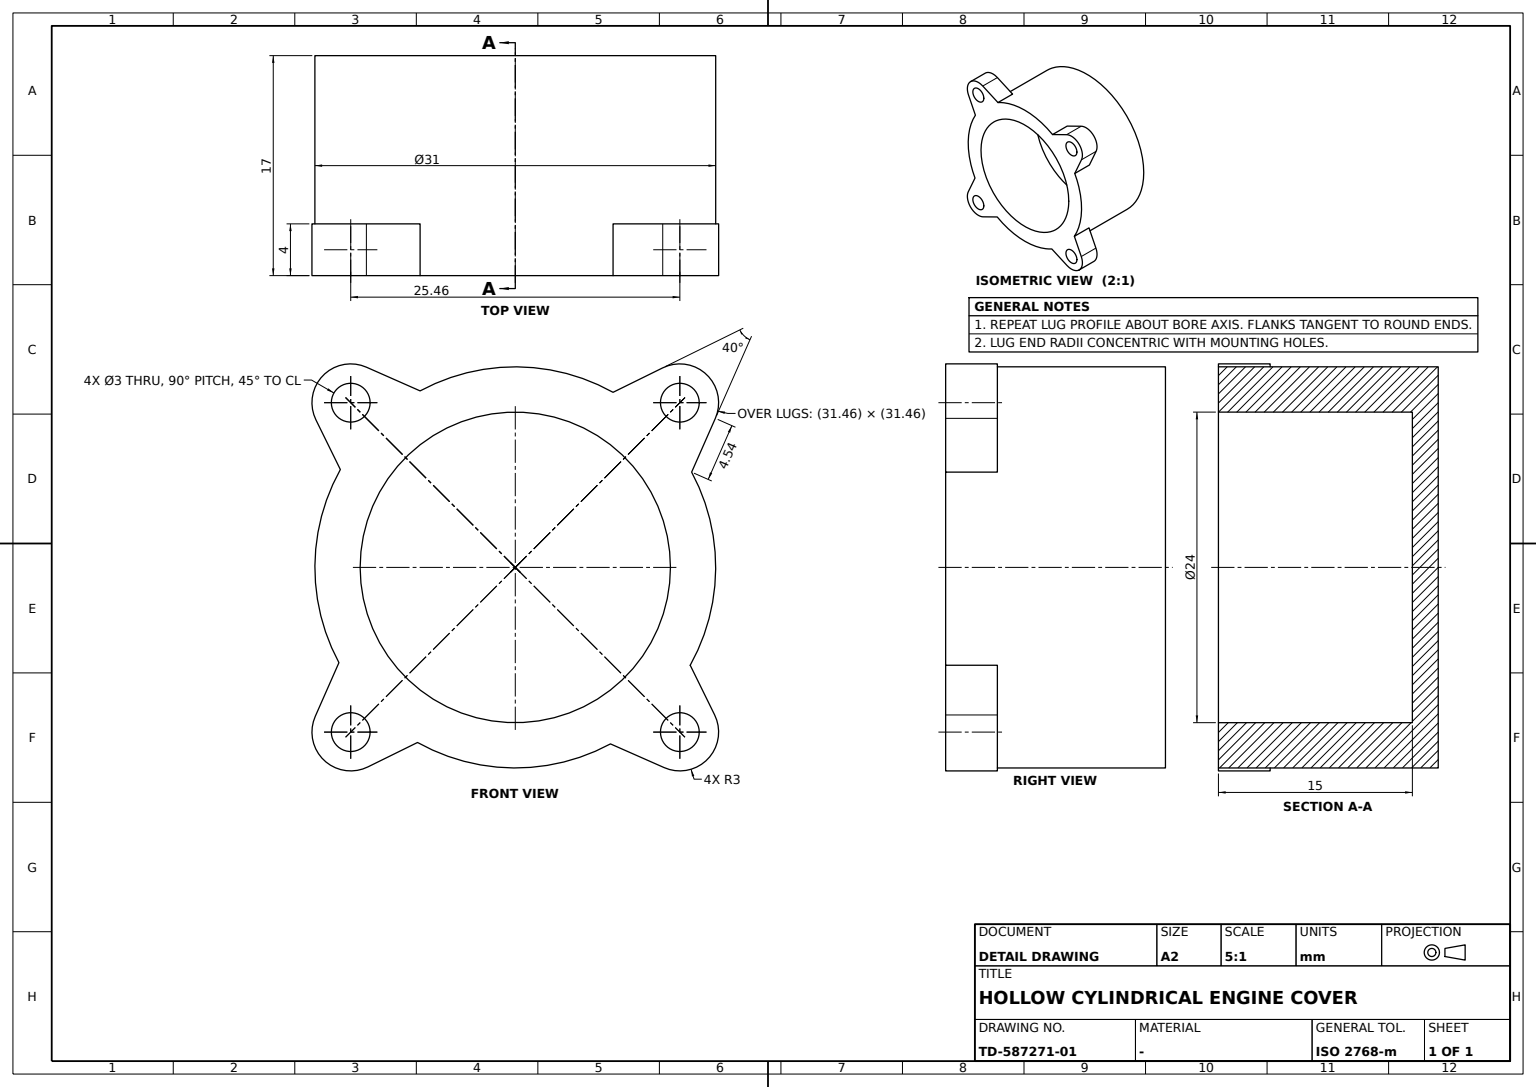
ISO-10303-21;
HEADER;
FILE_DESCRIPTION((''),'2;1');
FILE_NAME('','',(''),(''),'','','');
FILE_SCHEMA(('AUTOMOTIVE_DESIGN'));
ENDSEC;
DATA;
#1=APPLICATION_CONTEXT('');
#2=PRODUCT_CONTEXT('',#1,'mechanical');
#3=PRODUCT('','','',(#2));
#4=PRODUCT_DEFINITION_FORMATION('','',#3);
#5=PRODUCT_DEFINITION_CONTEXT('',#1,'design');
#6=PRODUCT_DEFINITION('','',#4,#5);
#7=PRODUCT_DEFINITION_SHAPE('','',#6);
#8=(LENGTH_UNIT()NAMED_UNIT(*)SI_UNIT(.MILLI.,.METRE.));
#9=(NAMED_UNIT(*)PLANE_ANGLE_UNIT()SI_UNIT($,.RADIAN.));
#10=(NAMED_UNIT(*)SI_UNIT($,.STERADIAN.)SOLID_ANGLE_UNIT());
#11=UNCERTAINTY_MEASURE_WITH_UNIT(LENGTH_MEASURE(0.005),#8,'distance_accuracy_value','');
#12=(GEOMETRIC_REPRESENTATION_CONTEXT(3)GLOBAL_UNCERTAINTY_ASSIGNED_CONTEXT((#11))GLOBAL_UNIT_ASSIGNED_CONTEXT((#8,#9,#10))REPRESENTATION_CONTEXT('',''));
#13=CARTESIAN_POINT('',(13.530058,-7.562244,13.));
#14=VERTEX_POINT('',#13);
#15=CARTESIAN_POINT('',(15.419817,-11.403653,13.));
#16=VERTEX_POINT('',#15);
#17=CARTESIAN_POINT('',(11.498549,-3.432692,13.));
#18=DIRECTION('',(0.441421476,-0.897299883,0.));
#19=VECTOR('',#18,1000.);
#20=LINE('',#17,#19);
#21=EDGE_CURVE('',#14,#16,#20,.T.);
#22=ORIENTED_EDGE('',*,*,#21,.T.);
#23=CARTESIAN_POINT('',(11.517023,-15.472682,13.));
#24=VERTEX_POINT('',#23);
#25=CARTESIAN_POINT('',(12.727917,-12.727917,13.));
#26=DIRECTION('',(0.,0.,1.));
#27=DIRECTION('',(1.,0.,0.));
#28=AXIS2_PLACEMENT_3D('',#25,#26,#27);
#29=CIRCLE('',#28,3.);
#30=EDGE_CURVE('',#24,#16,#29,.T.);
#31=ORIENTED_EDGE('',*,*,#30,.F.);
#32=CARTESIAN_POINT('',(7.362426,-13.63982,13.));
#33=VERTEX_POINT('',#32);
#34=DIRECTION('',(-0.914921716,0.403631334,0.));
#35=VECTOR('',#34,1000.);
#36=LINE('',#23,#35);
#37=EDGE_CURVE('',#24,#33,#36,.T.);
#38=ORIENTED_EDGE('',*,*,#37,.T.);
#39=CARTESIAN_POINT('',(0.,0.,13.));
#40=AXIS2_PLACEMENT_3D('',#39,#26,#27);
#41=CIRCLE('',#40,15.5);
#42=EDGE_CURVE('',#33,#14,#41,.T.);
#43=ORIENTED_EDGE('',*,*,#42,.T.);
#44=EDGE_LOOP('',(#22,#31,#38,#43));
#45=FACE_BOUND('',#44,.T.);
#46=CARTESIAN_POINT('',(14.227917,-12.727917,13.));
#47=VERTEX_POINT('',#46);
#48=CIRCLE('',#28,1.5);
#49=EDGE_CURVE('',#47,#47,#48,.T.);
#50=ORIENTED_EDGE('',*,*,#49,.T.);
#51=EDGE_LOOP('',(#50));
#52=FACE_BOUND('',#51,.T.);
#53=DIRECTION('',(0.,1.,0.));
#54=AXIS2_PLACEMENT_3D('',#39,#26,#53);
#55=PLANE('',#54);
#56=ADVANCED_FACE('',(#45,#52),#55,.F.);
#57=CARTESIAN_POINT('',(-13.63982,-7.362426,17.));
#58=VERTEX_POINT('',#57);
#59=CARTESIAN_POINT('',(-13.63982,-7.362426,13.));
#60=VERTEX_POINT('',#59);
#61=VECTOR('',#26,1000.);
#62=LINE('',#57,#61);
#63=EDGE_CURVE('',#58,#60,#62,.F.);
#64=ORIENTED_EDGE('',*,*,#63,.T.);
#65=CARTESIAN_POINT('',(-15.472682,-11.517023,13.));
#66=VERTEX_POINT('',#65);
#67=DIRECTION('',(0.403631334,0.914921716,0.));
#68=VECTOR('',#67,1000.);
#69=LINE('',#65,#68);
#70=EDGE_CURVE('',#66,#60,#69,.T.);
#71=ORIENTED_EDGE('',*,*,#70,.F.);
#72=CARTESIAN_POINT('',(-15.472682,-11.517023,17.));
#73=VERTEX_POINT('',#72);
#74=CARTESIAN_POINT('',(-15.472682,-11.517023,15.));
#75=LINE('',#74,#61);
#76=EDGE_CURVE('',#73,#66,#75,.F.);
#77=ORIENTED_EDGE('',*,*,#76,.F.);
#78=LINE('',#72,#68);
#79=EDGE_CURVE('',#73,#58,#78,.T.);
#80=ORIENTED_EDGE('',*,*,#79,.T.);
#81=EDGE_LOOP('',(#64,#71,#77,#80));
#82=FACE_BOUND('',#81,.T.);
#83=AXIS2_PLACEMENT_3D('',#72,#34,#67);
#84=PLANE('',#83);
#85=ADVANCED_FACE('',(#82),#84,.T.);
#86=CARTESIAN_POINT('',(-11.517023,15.472682,17.));
#87=VERTEX_POINT('',#86);
#88=CARTESIAN_POINT('',(-11.517023,15.472682,13.));
#89=VERTEX_POINT('',#88);
#90=CARTESIAN_POINT('',(-11.517023,15.472682,15.));
#91=LINE('',#90,#61);
#92=EDGE_CURVE('',#87,#89,#91,.F.);
#93=ORIENTED_EDGE('',*,*,#92,.F.);
#94=CARTESIAN_POINT('',(-7.362426,13.63982,17.));
#95=VERTEX_POINT('',#94);
#96=DIRECTION('',(0.914921716,-0.403631334,0.));
#97=VECTOR('',#96,1000.);
#98=LINE('',#86,#97);
#99=EDGE_CURVE('',#87,#95,#98,.T.);
#100=ORIENTED_EDGE('',*,*,#99,.T.);
#101=CARTESIAN_POINT('',(-7.362426,13.63982,13.));
#102=VERTEX_POINT('',#101);
#103=LINE('',#94,#61);
#104=EDGE_CURVE('',#95,#102,#103,.F.);
#105=ORIENTED_EDGE('',*,*,#104,.T.);
#106=LINE('',#88,#97);
#107=EDGE_CURVE('',#89,#102,#106,.T.);
#108=ORIENTED_EDGE('',*,*,#107,.F.);
#109=EDGE_LOOP('',(#93,#100,#105,#108));
#110=FACE_BOUND('',#109,.T.);
#111=AXIS2_PLACEMENT_3D('',#86,#67,#96);
#112=PLANE('',#111);
#113=ADVANCED_FACE('',(#110),#112,.T.);
#114=CARTESIAN_POINT('',(-11.403653,-15.419817,17.));
#115=VERTEX_POINT('',#114);
#116=CARTESIAN_POINT('',(-12.727917,-12.727917,17.));
#117=AXIS2_PLACEMENT_3D('',#116,#26,#27);
#118=CIRCLE('',#117,3.);
#119=EDGE_CURVE('',#73,#115,#118,.T.);
#120=ORIENTED_EDGE('',*,*,#119,.F.);
#121=ORIENTED_EDGE('',*,*,#76,.T.);
#122=CARTESIAN_POINT('',(-11.403653,-15.419817,13.));
#123=VERTEX_POINT('',#122);
#124=CARTESIAN_POINT('',(-12.727917,-12.727917,13.));
#125=AXIS2_PLACEMENT_3D('',#124,#26,#27);
#126=CIRCLE('',#125,3.);
#127=EDGE_CURVE('',#66,#123,#126,.T.);
#128=ORIENTED_EDGE('',*,*,#127,.T.);
#129=CARTESIAN_POINT('',(-11.403653,-15.419817,15.));
#130=LINE('',#129,#61);
#131=EDGE_CURVE('',#115,#123,#130,.F.);
#132=ORIENTED_EDGE('',*,*,#131,.F.);
#133=EDGE_LOOP('',(#120,#121,#128,#132));
#134=FACE_BOUND('',#133,.T.);
#135=CARTESIAN_POINT('',(-12.727917,-12.727917,15.));
#136=DIRECTION('',(-1.,0.,0.));
#137=AXIS2_PLACEMENT_3D('',#135,#26,#136);
#138=CYLINDRICAL_SURFACE('',#137,3.);
#139=ADVANCED_FACE('',(#134),#138,.T.);
#140=CARTESIAN_POINT('',(11.517023,-15.472682,17.));
#141=VERTEX_POINT('',#140);
#142=CARTESIAN_POINT('',(11.517023,-15.472682,15.));
#143=LINE('',#142,#61);
#144=EDGE_CURVE('',#141,#24,#143,.F.);
#145=ORIENTED_EDGE('',*,*,#144,.F.);
#146=CARTESIAN_POINT('',(7.362426,-13.63982,17.));
#147=VERTEX_POINT('',#146);
#148=LINE('',#140,#35);
#149=EDGE_CURVE('',#141,#147,#148,.T.);
#150=ORIENTED_EDGE('',*,*,#149,.T.);
#151=LINE('',#146,#61);
#152=EDGE_CURVE('',#147,#33,#151,.F.);
#153=ORIENTED_EDGE('',*,*,#152,.T.);
#154=ORIENTED_EDGE('',*,*,#37,.F.);
#155=EDGE_LOOP('',(#145,#150,#153,#154));
#156=FACE_BOUND('',#155,.T.);
#157=DIRECTION('',(-0.403631334,-0.914921716,0.));
#158=AXIS2_PLACEMENT_3D('',#140,#157,#34);
#159=PLANE('',#158);
#160=ADVANCED_FACE('',(#156),#159,.T.);
#161=CARTESIAN_POINT('',(7.562244,13.530058,13.));
#162=VERTEX_POINT('',#161);
#163=CARTESIAN_POINT('',(11.403653,15.419817,13.));
#164=VERTEX_POINT('',#163);
#165=CARTESIAN_POINT('',(3.432692,11.498549,13.));
#166=DIRECTION('',(0.897299883,0.441421476,0.));
#167=VECTOR('',#166,1000.);
#168=LINE('',#165,#167);
#169=EDGE_CURVE('',#162,#164,#168,.T.);
#170=ORIENTED_EDGE('',*,*,#169,.F.);
#171=CARTESIAN_POINT('',(7.562244,13.530058,17.));
#172=VERTEX_POINT('',#171);
#173=LINE('',#171,#61);
#174=EDGE_CURVE('',#172,#162,#173,.F.);
#175=ORIENTED_EDGE('',*,*,#174,.F.);
#176=CARTESIAN_POINT('',(11.403653,15.419817,17.));
#177=VERTEX_POINT('',#176);
#178=CARTESIAN_POINT('',(3.432692,11.498549,17.));
#179=LINE('',#178,#167);
#180=EDGE_CURVE('',#172,#177,#179,.T.);
#181=ORIENTED_EDGE('',*,*,#180,.T.);
#182=CARTESIAN_POINT('',(11.403653,15.419817,15.));
#183=LINE('',#182,#61);
#184=EDGE_CURVE('',#177,#164,#183,.F.);
#185=ORIENTED_EDGE('',*,*,#184,.T.);
#186=EDGE_LOOP('',(#170,#175,#181,#185));
#187=FACE_BOUND('',#186,.T.);
#188=DIRECTION('',(-0.441421476,0.897299883,0.));
#189=AXIS2_PLACEMENT_3D('',#178,#188,#166);
#190=PLANE('',#189);
#191=ADVANCED_FACE('',(#187),#190,.T.);
#192=CARTESIAN_POINT('',(15.472682,11.517023,17.));
#193=VERTEX_POINT('',#192);
#194=CARTESIAN_POINT('',(12.727917,12.727917,17.));
#195=AXIS2_PLACEMENT_3D('',#194,#26,#27);
#196=CIRCLE('',#195,3.);
#197=EDGE_CURVE('',#193,#177,#196,.T.);
#198=ORIENTED_EDGE('',*,*,#197,.F.);
#199=CARTESIAN_POINT('',(15.472682,11.517023,13.));
#200=VERTEX_POINT('',#199);
#201=CARTESIAN_POINT('',(15.472682,11.517023,15.));
#202=LINE('',#201,#61);
#203=EDGE_CURVE('',#193,#200,#202,.F.);
#204=ORIENTED_EDGE('',*,*,#203,.T.);
#205=CARTESIAN_POINT('',(12.727917,12.727917,13.));
#206=AXIS2_PLACEMENT_3D('',#205,#26,#27);
#207=CIRCLE('',#206,3.);
#208=EDGE_CURVE('',#200,#164,#207,.T.);
#209=ORIENTED_EDGE('',*,*,#208,.T.);
#210=ORIENTED_EDGE('',*,*,#184,.F.);
#211=EDGE_LOOP('',(#198,#204,#209,#210));
#212=FACE_BOUND('',#211,.T.);
#213=CARTESIAN_POINT('',(12.727917,12.727917,15.));
#214=AXIS2_PLACEMENT_3D('',#213,#26,#27);
#215=CYLINDRICAL_SURFACE('',#214,3.);
#216=ADVANCED_FACE('',(#212),#215,.T.);
#217=CARTESIAN_POINT('',(-11.227917,12.727917,13.));
#218=VERTEX_POINT('',#217);
#219=CARTESIAN_POINT('',(-12.727917,12.727917,13.));
#220=AXIS2_PLACEMENT_3D('',#219,#26,#27);
#221=CIRCLE('',#220,1.5);
#222=EDGE_CURVE('',#218,#218,#221,.T.);
#223=ORIENTED_EDGE('',*,*,#222,.T.);
#224=EDGE_LOOP('',(#223));
#225=FACE_BOUND('',#224,.T.);
#226=CARTESIAN_POINT('',(-13.530058,7.562244,13.));
#227=VERTEX_POINT('',#226);
#228=EDGE_CURVE('',#102,#227,#41,.T.);
#229=ORIENTED_EDGE('',*,*,#228,.T.);
#230=CARTESIAN_POINT('',(-15.419817,11.403653,13.));
#231=VERTEX_POINT('',#230);
#232=CARTESIAN_POINT('',(-11.498549,3.432692,13.));
#233=VECTOR('',#188,1000.);
#234=LINE('',#232,#233);
#235=EDGE_CURVE('',#227,#231,#234,.T.);
#236=ORIENTED_EDGE('',*,*,#235,.T.);
#237=CIRCLE('',#220,3.);
#238=EDGE_CURVE('',#89,#231,#237,.T.);
#239=ORIENTED_EDGE('',*,*,#238,.F.);
#240=ORIENTED_EDGE('',*,*,#107,.T.);
#241=EDGE_LOOP('',(#229,#236,#239,#240));
#242=FACE_BOUND('',#241,.T.);
#243=ADVANCED_FACE('',(#225,#242),#55,.F.);
#244=CARTESIAN_POINT('',(-15.419817,11.403653,17.));
#245=VERTEX_POINT('',#244);
#246=CARTESIAN_POINT('',(-12.727917,12.727917,17.));
#247=AXIS2_PLACEMENT_3D('',#246,#26,#27);
#248=CIRCLE('',#247,3.);
#249=EDGE_CURVE('',#87,#245,#248,.T.);
#250=ORIENTED_EDGE('',*,*,#249,.F.);
#251=ORIENTED_EDGE('',*,*,#92,.T.);
#252=ORIENTED_EDGE('',*,*,#238,.T.);
#253=CARTESIAN_POINT('',(-15.419817,11.403653,15.));
#254=LINE('',#253,#61);
#255=EDGE_CURVE('',#245,#231,#254,.F.);
#256=ORIENTED_EDGE('',*,*,#255,.F.);
#257=EDGE_LOOP('',(#250,#251,#252,#256));
#258=FACE_BOUND('',#257,.T.);
#259=CARTESIAN_POINT('',(-12.727917,12.727917,15.));
#260=AXIS2_PLACEMENT_3D('',#259,#26,#53);
#261=CYLINDRICAL_SURFACE('',#260,3.);
#262=ADVANCED_FACE('',(#258),#261,.T.);
#263=CARTESIAN_POINT('',(13.530058,-7.562244,17.));
#264=VERTEX_POINT('',#263);
#265=LINE('',#263,#61);
#266=EDGE_CURVE('',#264,#14,#265,.F.);
#267=ORIENTED_EDGE('',*,*,#266,.F.);
#268=CARTESIAN_POINT('',(15.419817,-11.403653,17.));
#269=VERTEX_POINT('',#268);
#270=CARTESIAN_POINT('',(11.498549,-3.432692,17.));
#271=LINE('',#270,#19);
#272=EDGE_CURVE('',#264,#269,#271,.T.);
#273=ORIENTED_EDGE('',*,*,#272,.T.);
#274=CARTESIAN_POINT('',(15.419817,-11.403653,15.));
#275=LINE('',#274,#61);
#276=EDGE_CURVE('',#269,#16,#275,.F.);
#277=ORIENTED_EDGE('',*,*,#276,.T.);
#278=ORIENTED_EDGE('',*,*,#21,.F.);
#279=EDGE_LOOP('',(#267,#273,#277,#278));
#280=FACE_BOUND('',#279,.T.);
#281=AXIS2_PLACEMENT_3D('',#270,#166,#18);
#282=PLANE('',#281);
#283=ADVANCED_FACE('',(#280),#282,.T.);
#284=CARTESIAN_POINT('',(13.63982,7.362426,17.));
#285=VERTEX_POINT('',#284);
#286=VECTOR('',#157,1000.);
#287=LINE('',#192,#286);
#288=EDGE_CURVE('',#193,#285,#287,.T.);
#289=ORIENTED_EDGE('',*,*,#288,.T.);
#290=CARTESIAN_POINT('',(13.63982,7.362426,13.));
#291=VERTEX_POINT('',#290);
#292=LINE('',#284,#61);
#293=EDGE_CURVE('',#285,#291,#292,.F.);
#294=ORIENTED_EDGE('',*,*,#293,.T.);
#295=LINE('',#199,#286);
#296=EDGE_CURVE('',#200,#291,#295,.T.);
#297=ORIENTED_EDGE('',*,*,#296,.F.);
#298=ORIENTED_EDGE('',*,*,#203,.F.);
#299=EDGE_LOOP('',(#289,#294,#297,#298));
#300=FACE_BOUND('',#299,.T.);
#301=AXIS2_PLACEMENT_3D('',#192,#96,#157);
#302=PLANE('',#301);
#303=ADVANCED_FACE('',(#300),#302,.T.);
#304=CARTESIAN_POINT('',(14.227917,12.727917,13.));
#305=VERTEX_POINT('',#304);
#306=CIRCLE('',#206,1.5);
#307=EDGE_CURVE('',#305,#305,#306,.T.);
#308=ORIENTED_EDGE('',*,*,#307,.T.);
#309=EDGE_LOOP('',(#308));
#310=FACE_BOUND('',#309,.T.);
#311=ORIENTED_EDGE('',*,*,#169,.T.);
#312=ORIENTED_EDGE('',*,*,#208,.F.);
#313=ORIENTED_EDGE('',*,*,#296,.T.);
#314=EDGE_CURVE('',#291,#162,#41,.T.);
#315=ORIENTED_EDGE('',*,*,#314,.T.);
#316=EDGE_LOOP('',(#311,#312,#313,#315));
#317=FACE_BOUND('',#316,.T.);
#318=ADVANCED_FACE('',(#310,#317),#55,.F.);
#319=CARTESIAN_POINT('',(12.,0.,17.));
#320=VERTEX_POINT('',#319);
#321=CARTESIAN_POINT('',(0.,0.,17.));
#322=AXIS2_PLACEMENT_3D('',#321,#26,#27);
#323=CIRCLE('',#322,12.);
#324=EDGE_CURVE('',#320,#320,#323,.T.);
#325=ORIENTED_EDGE('',*,*,#324,.T.);
#326=EDGE_LOOP('',(#325));
#327=FACE_BOUND('',#326,.T.);
#328=CARTESIAN_POINT('',(12.,0.,2.));
#329=VERTEX_POINT('',#328);
#330=CARTESIAN_POINT('',(0.,0.,2.));
#331=AXIS2_PLACEMENT_3D('',#330,#26,#27);
#332=CIRCLE('',#331,12.);
#333=EDGE_CURVE('',#329,#329,#332,.T.);
#334=ORIENTED_EDGE('',*,*,#333,.F.);
#335=EDGE_LOOP('',(#334));
#336=FACE_BOUND('',#335,.T.);
#337=CARTESIAN_POINT('',(0.,0.,9.5));
#338=AXIS2_PLACEMENT_3D('',#337,#26,#27);
#339=CYLINDRICAL_SURFACE('',#338,12.);
#340=ADVANCED_FACE('',(#327,#336),#339,.F.);
#341=CARTESIAN_POINT('',(-11.227917,-12.727917,17.));
#342=VERTEX_POINT('',#341);
#343=CIRCLE('',#117,1.5);
#344=EDGE_CURVE('',#342,#342,#343,.T.);
#345=ORIENTED_EDGE('',*,*,#344,.T.);
#346=EDGE_LOOP('',(#345));
#347=FACE_BOUND('',#346,.T.);
#348=CARTESIAN_POINT('',(-11.227917,-12.727917,13.));
#349=VERTEX_POINT('',#348);
#350=CIRCLE('',#125,1.5);
#351=EDGE_CURVE('',#349,#349,#350,.T.);
#352=ORIENTED_EDGE('',*,*,#351,.F.);
#353=EDGE_LOOP('',(#352));
#354=FACE_BOUND('',#353,.T.);
#355=CYLINDRICAL_SURFACE('',#137,1.5);
#356=ADVANCED_FACE('',(#347,#354),#355,.F.);
#357=ORIENTED_EDGE('',*,*,#324,.F.);
#358=EDGE_LOOP('',(#357));
#359=FACE_BOUND('',#358,.T.);
#360=CARTESIAN_POINT('',(-11.227917,12.727917,17.));
#361=VERTEX_POINT('',#360);
#362=CIRCLE('',#247,1.5);
#363=EDGE_CURVE('',#361,#361,#362,.T.);
#364=ORIENTED_EDGE('',*,*,#363,.F.);
#365=EDGE_LOOP('',(#364));
#366=FACE_BOUND('',#365,.T.);
#367=ORIENTED_EDGE('',*,*,#344,.F.);
#368=EDGE_LOOP('',(#367));
#369=FACE_BOUND('',#368,.T.);
#370=CARTESIAN_POINT('',(14.227917,12.727917,17.));
#371=VERTEX_POINT('',#370);
#372=CIRCLE('',#195,1.5);
#373=EDGE_CURVE('',#371,#371,#372,.T.);
#374=ORIENTED_EDGE('',*,*,#373,.F.);
#375=EDGE_LOOP('',(#374));
#376=FACE_BOUND('',#375,.T.);
#377=CARTESIAN_POINT('',(-7.562244,-13.530058,17.));
#378=VERTEX_POINT('',#377);
#379=CARTESIAN_POINT('',(-3.432692,-11.498549,17.));
#380=DIRECTION('',(-0.897299883,-0.441421476,0.));
#381=VECTOR('',#380,1000.);
#382=LINE('',#379,#381);
#383=EDGE_CURVE('',#378,#115,#382,.T.);
#384=ORIENTED_EDGE('',*,*,#383,.F.);
#385=CIRCLE('',#322,15.5);
#386=EDGE_CURVE('',#378,#147,#385,.T.);
#387=ORIENTED_EDGE('',*,*,#386,.T.);
#388=ORIENTED_EDGE('',*,*,#149,.F.);
#389=CARTESIAN_POINT('',(12.727917,-12.727917,17.));
#390=AXIS2_PLACEMENT_3D('',#389,#26,#27);
#391=CIRCLE('',#390,3.);
#392=EDGE_CURVE('',#141,#269,#391,.T.);
#393=ORIENTED_EDGE('',*,*,#392,.T.);
#394=ORIENTED_EDGE('',*,*,#272,.F.);
#395=EDGE_CURVE('',#264,#285,#385,.T.);
#396=ORIENTED_EDGE('',*,*,#395,.T.);
#397=ORIENTED_EDGE('',*,*,#288,.F.);
#398=ORIENTED_EDGE('',*,*,#197,.T.);
#399=ORIENTED_EDGE('',*,*,#180,.F.);
#400=EDGE_CURVE('',#172,#95,#385,.T.);
#401=ORIENTED_EDGE('',*,*,#400,.T.);
#402=ORIENTED_EDGE('',*,*,#99,.F.);
#403=ORIENTED_EDGE('',*,*,#249,.T.);
#404=CARTESIAN_POINT('',(-13.530058,7.562244,17.));
#405=VERTEX_POINT('',#404);
#406=CARTESIAN_POINT('',(-11.498549,3.432692,17.));
#407=LINE('',#406,#233);
#408=EDGE_CURVE('',#405,#245,#407,.T.);
#409=ORIENTED_EDGE('',*,*,#408,.F.);
#410=EDGE_CURVE('',#405,#58,#385,.T.);
#411=ORIENTED_EDGE('',*,*,#410,.T.);
#412=ORIENTED_EDGE('',*,*,#79,.F.);
#413=ORIENTED_EDGE('',*,*,#119,.T.);
#414=EDGE_LOOP('',(#384,#387,#388,#393,#394,#396,#397,#398,#399,#401,#402,#403,#409,#411,#412,#413));
#415=FACE_BOUND('',#414,.T.);
#416=CARTESIAN_POINT('',(14.227917,-12.727917,17.));
#417=VERTEX_POINT('',#416);
#418=CIRCLE('',#390,1.5);
#419=EDGE_CURVE('',#417,#417,#418,.T.);
#420=ORIENTED_EDGE('',*,*,#419,.F.);
#421=EDGE_LOOP('',(#420));
#422=FACE_BOUND('',#421,.T.);
#423=AXIS2_PLACEMENT_3D('',#321,#26,#53);
#424=PLANE('',#423);
#425=ADVANCED_FACE('',(#359,#366,#369,#376,#415,#422),#424,.T.);
#426=ORIENTED_EDGE('',*,*,#307,.F.);
#427=EDGE_LOOP('',(#426));
#428=FACE_BOUND('',#427,.T.);
#429=ORIENTED_EDGE('',*,*,#373,.T.);
#430=EDGE_LOOP('',(#429));
#431=FACE_BOUND('',#430,.T.);
#432=CYLINDRICAL_SURFACE('',#214,1.5);
#433=ADVANCED_FACE('',(#428,#431),#432,.F.);
#434=ORIENTED_EDGE('',*,*,#383,.T.);
#435=ORIENTED_EDGE('',*,*,#131,.T.);
#436=CARTESIAN_POINT('',(-7.562244,-13.530058,13.));
#437=VERTEX_POINT('',#436);
#438=CARTESIAN_POINT('',(-3.432692,-11.498549,13.));
#439=LINE('',#438,#381);
#440=EDGE_CURVE('',#437,#123,#439,.T.);
#441=ORIENTED_EDGE('',*,*,#440,.F.);
#442=LINE('',#377,#61);
#443=EDGE_CURVE('',#378,#437,#442,.F.);
#444=ORIENTED_EDGE('',*,*,#443,.F.);
#445=EDGE_LOOP('',(#434,#435,#441,#444));
#446=FACE_BOUND('',#445,.T.);
#447=AXIS2_PLACEMENT_3D('',#379,#18,#380);
#448=PLANE('',#447);
#449=ADVANCED_FACE('',(#446),#448,.T.);
#450=ORIENTED_EDGE('',*,*,#363,.T.);
#451=EDGE_LOOP('',(#450));
#452=FACE_BOUND('',#451,.T.);
#453=ORIENTED_EDGE('',*,*,#222,.F.);
#454=EDGE_LOOP('',(#453));
#455=FACE_BOUND('',#454,.T.);
#456=CYLINDRICAL_SURFACE('',#260,1.5);
#457=ADVANCED_FACE('',(#452,#455),#456,.F.);
#458=ORIENTED_EDGE('',*,*,#49,.F.);
#459=EDGE_LOOP('',(#458));
#460=FACE_BOUND('',#459,.T.);
#461=ORIENTED_EDGE('',*,*,#419,.T.);
#462=EDGE_LOOP('',(#461));
#463=FACE_BOUND('',#462,.T.);
#464=CARTESIAN_POINT('',(12.727917,-12.727917,15.));
#465=DIRECTION('',(0.,-1.,0.));
#466=AXIS2_PLACEMENT_3D('',#464,#26,#465);
#467=CYLINDRICAL_SURFACE('',#466,1.5);
#468=ADVANCED_FACE('',(#460,#463),#467,.F.);
#469=CARTESIAN_POINT('',(15.5,0.,0.));
#470=VERTEX_POINT('',#469);
#471=CARTESIAN_POINT('',(0.,0.,0.));
#472=AXIS2_PLACEMENT_3D('',#471,#26,#27);
#473=CIRCLE('',#472,15.5);
#474=EDGE_CURVE('',#470,#470,#473,.T.);
#475=ORIENTED_EDGE('',*,*,#474,.F.);
#476=EDGE_LOOP('',(#475));
#477=FACE_BOUND('',#476,.T.);
#478=AXIS2_PLACEMENT_3D('',#471,#26,#53);
#479=PLANE('',#478);
#480=ADVANCED_FACE('',(#477),#479,.F.);
#481=ORIENTED_EDGE('',*,*,#440,.T.);
#482=ORIENTED_EDGE('',*,*,#127,.F.);
#483=ORIENTED_EDGE('',*,*,#70,.T.);
#484=EDGE_CURVE('',#60,#437,#41,.T.);
#485=ORIENTED_EDGE('',*,*,#484,.T.);
#486=EDGE_LOOP('',(#481,#482,#483,#485));
#487=FACE_BOUND('',#486,.T.);
#488=ORIENTED_EDGE('',*,*,#351,.T.);
#489=EDGE_LOOP('',(#488));
#490=FACE_BOUND('',#489,.T.);
#491=ADVANCED_FACE('',(#487,#490),#55,.F.);
#492=ORIENTED_EDGE('',*,*,#333,.T.);
#493=EDGE_LOOP('',(#492));
#494=FACE_BOUND('',#493,.T.);
#495=PLANE('',#331);
#496=ADVANCED_FACE('',(#494),#495,.T.);
#497=ORIENTED_EDGE('',*,*,#235,.F.);
#498=LINE('',#404,#61);
#499=EDGE_CURVE('',#405,#227,#498,.F.);
#500=ORIENTED_EDGE('',*,*,#499,.F.);
#501=ORIENTED_EDGE('',*,*,#408,.T.);
#502=ORIENTED_EDGE('',*,*,#255,.T.);
#503=EDGE_LOOP('',(#497,#500,#501,#502));
#504=FACE_BOUND('',#503,.T.);
#505=AXIS2_PLACEMENT_3D('',#406,#380,#188);
#506=PLANE('',#505);
#507=ADVANCED_FACE('',(#504),#506,.T.);
#508=ORIENTED_EDGE('',*,*,#266,.T.);
#509=ORIENTED_EDGE('',*,*,#42,.F.);
#510=ORIENTED_EDGE('',*,*,#152,.F.);
#511=ORIENTED_EDGE('',*,*,#386,.F.);
#512=ORIENTED_EDGE('',*,*,#443,.T.);
#513=ORIENTED_EDGE('',*,*,#484,.F.);
#514=ORIENTED_EDGE('',*,*,#63,.F.);
#515=ORIENTED_EDGE('',*,*,#410,.F.);
#516=ORIENTED_EDGE('',*,*,#499,.T.);
#517=ORIENTED_EDGE('',*,*,#228,.F.);
#518=ORIENTED_EDGE('',*,*,#104,.F.);
#519=ORIENTED_EDGE('',*,*,#400,.F.);
#520=ORIENTED_EDGE('',*,*,#174,.T.);
#521=ORIENTED_EDGE('',*,*,#314,.F.);
#522=ORIENTED_EDGE('',*,*,#293,.F.);
#523=ORIENTED_EDGE('',*,*,#395,.F.);
#524=EDGE_LOOP('',(#508,#509,#510,#511,#512,#513,#514,#515,#516,#517,#518,#519,#520,#521,#522,#523));
#525=FACE_BOUND('',#524,.T.);
#526=ORIENTED_EDGE('',*,*,#474,.T.);
#527=EDGE_LOOP('',(#526));
#528=FACE_BOUND('',#527,.T.);
#529=CARTESIAN_POINT('',(0.,0.,8.5));
#530=AXIS2_PLACEMENT_3D('',#529,#26,#53);
#531=CYLINDRICAL_SURFACE('',#530,15.5);
#532=ADVANCED_FACE('',(#525,#528),#531,.T.);
#533=ORIENTED_EDGE('',*,*,#30,.T.);
#534=ORIENTED_EDGE('',*,*,#276,.F.);
#535=ORIENTED_EDGE('',*,*,#392,.F.);
#536=ORIENTED_EDGE('',*,*,#144,.T.);
#537=EDGE_LOOP('',(#533,#534,#535,#536));
#538=FACE_BOUND('',#537,.T.);
#539=CYLINDRICAL_SURFACE('',#466,3.);
#540=ADVANCED_FACE('',(#538),#539,.T.);
#541=CLOSED_SHELL('',(#56,#85,#113,#139,#160,#191,#216,#243,#262,#283,#303,#318,#340,#356,#425,#433,#449,#457,#468,#480,#491,#496,#507,#532,#540));
#542=MANIFOLD_SOLID_BREP('',#541);
#543=ADVANCED_BREP_SHAPE_REPRESENTATION('',(#542),#12);
#544=SHAPE_DEFINITION_REPRESENTATION(#7,#543);
ENDSEC;
END-ISO-10303-21;
